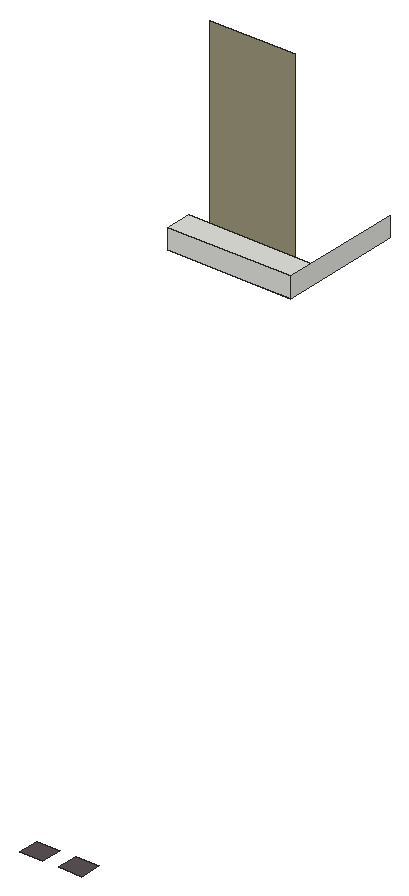
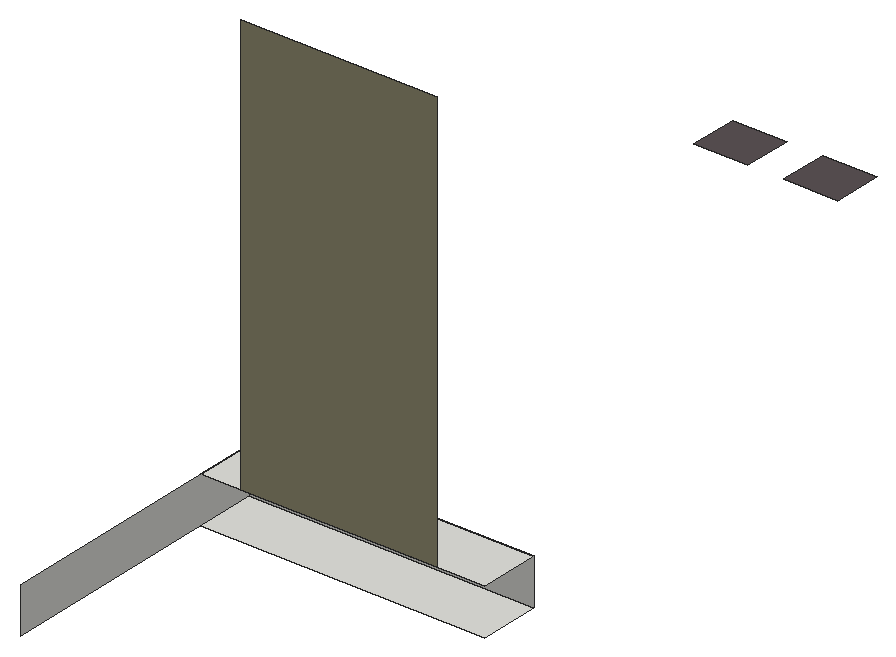
# SketchUp Ruby script. Lengths in inches.
U = 1.inch
M = Sketchup.active_model
def pt(a) = Geom::Point3d.new(a.map { |v| v * U })
def face(e, loops, mat)
  f = e.add_face(loops[0].map { |a| pt(a) })
  loops[1..].each { |l| e.add_face(l.map { |a| pt(a) }).erase! }
  f.material = f.back_material = mat if mat
  f
end
# faces: each face lists its corners as indices into pts; further lists are holes
def faces(e, pts, list, mat = nil) = list.each { |f| face(e, (f[0].is_a?(Array) ? f : [f]).map { |l| l.map { |i| pts[i] } }, mat) }
# xy, xz, yz: faces in a plane at the given z, y or x. An outline is a flat list of corners, or four numbers for a rectangle; further outlines are holes
def ring(l) = l.size == 4 ? [[l[0], l[1]], [l[2], l[1]], [l[2], l[3]], [l[0], l[3]]] : l.each_slice(2).to_a
def flat(e, list, mat, &to3) = list.each { |f| face(e, (f[0].is_a?(Array) ? f : [f]).map { |l| ring(l).map { |u, v| to3.(u, v) } }, mat) }
def xy(e, z, list, mat = nil) = flat(e, list, mat) { |x, y| [x, y, z] }
def xz(e, y, list, mat = nil) = flat(e, list, mat) { |x, z| [x, y, z] }
def yz(e, x, list, mat = nil) = flat(e, list, mat) { |y, z| [x, y, z] }
def lines(e, pts, list) = list.each { |a, b| e.add_line(pt(pts[a]), pt(pts[b])) }
# prism: a flat outline (further loops are holes) pulled along v
def prism(e, loops, v, mat = nil)
  f = face(e, loops, mat); d = Geom::Vector3d.new(v.map { |x| x * U })
  f.pushpull(f.normal.samedirection?(d) ? d.length : -d.length)
end
def box(e, o, s, mat = nil) = prism(e, [[o, [o[0] + s[0], o[1], o[2]], [o[0] + s[0], o[1] + s[1], o[2]], [o[0], o[1] + s[1], o[2]]]], [0, 0, s[2]], mat)
def at(x, y, z, deg = 0) = Geom::Transformation.translation(pt([x, y, z])) * Geom::Transformation.rotation(ORIGIN, Z_AXIS, deg.degrees)
def axes(o, x, y, z) = Geom::Transformation.new([*x, 0, *y, 0, *z, 0, *pt(o).to_a, 1])
def part(name) = M.definitions.add(name)
# library, detail: a bought-in or finely detailed component or shape, given as its bounding box
def library(name, o, s) = part(name).tap { |d| box(d.entities, o, s) }
def detail(e, o, s) = box(e.add_group.entities, o, s)
def put(e, d, t, mat = nil) = e.add_instance(d, t).tap { |i| i.material = mat if mat }
def group(e, t, mat = nil) = e.add_group.tap { |g| g.transformation = t; g.material = mat if mat }.entities
root = M.entities
M.materials.add("[Asphalt New]").color = [91, 82, 84]
M.materials.add("[Stone Coursed Rough]").color = [155, 150, 122]
xy(root,57.8125,[[334.81,92.3,339.17,96.24],[342.12,92.3,346.48,96.24]],"[Asphalt New]")
xy(root,92.87,[[277.93,198.23,301.1,203.17]])
xy(root,96.63,[[277.93,198.23,301.1,203.17]])
xz(root,198.23,[[277.93,92.87,301.1,96.63]])
xz(root,203.17,[[281.86,96.63,297.85,130.875]],"[Stone Coursed Rough]")
yz(root,301.1,[[198.23,92.87,221.48,96.63]])
